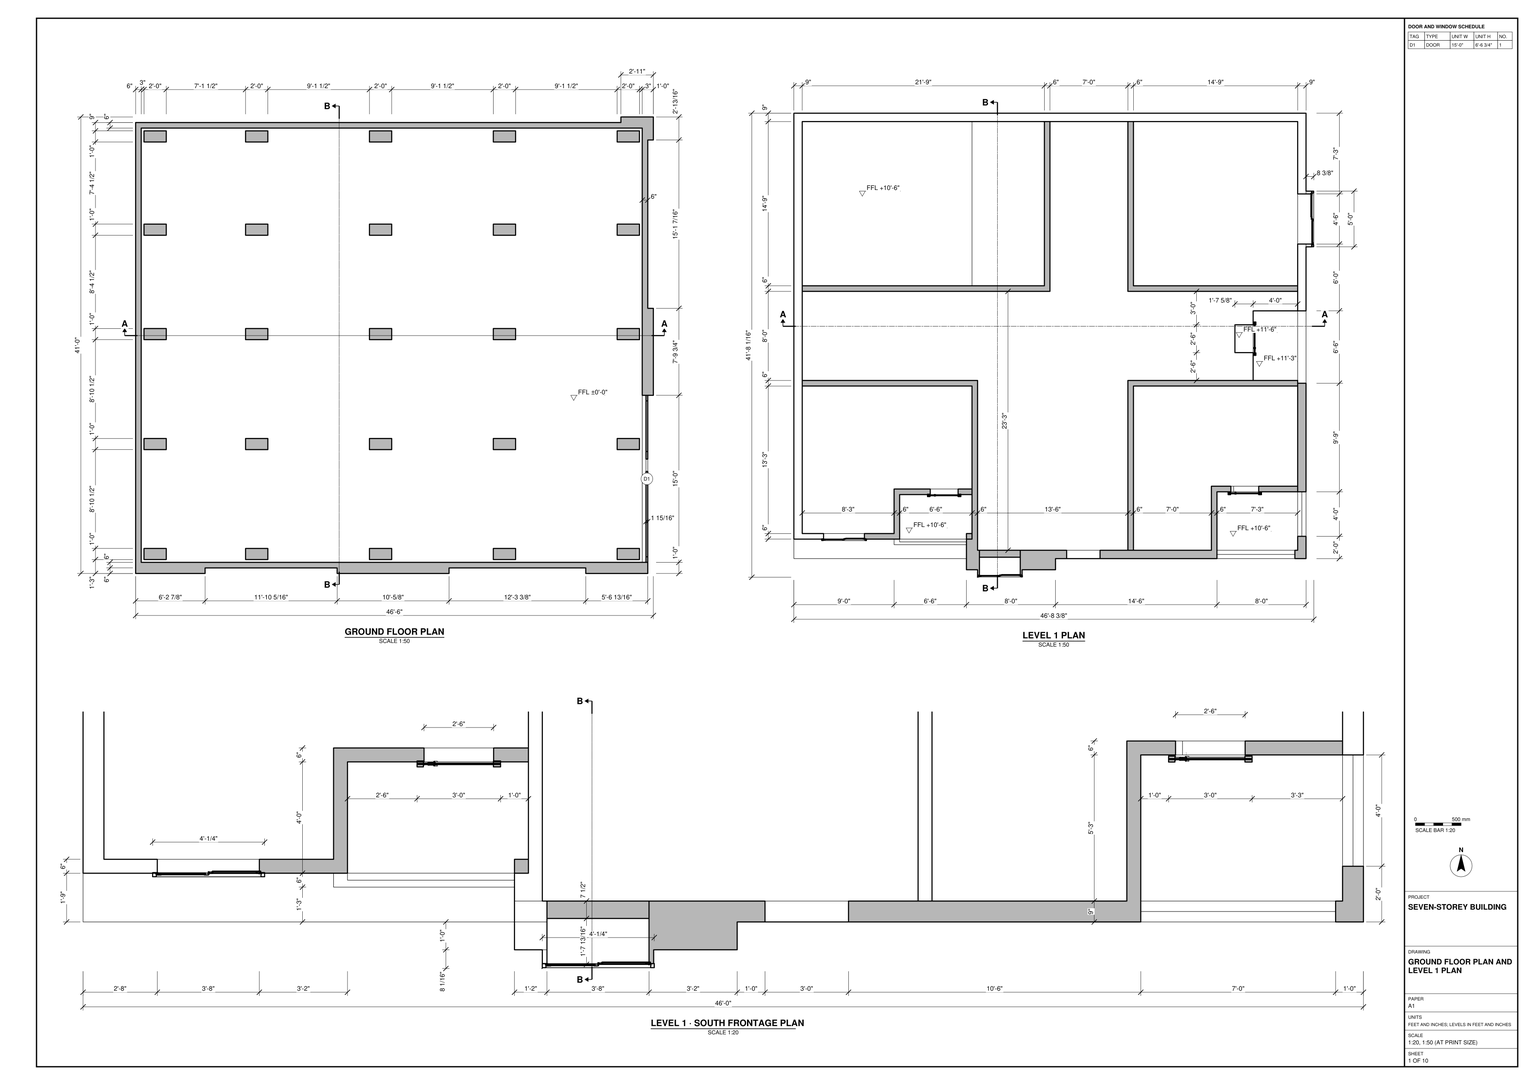
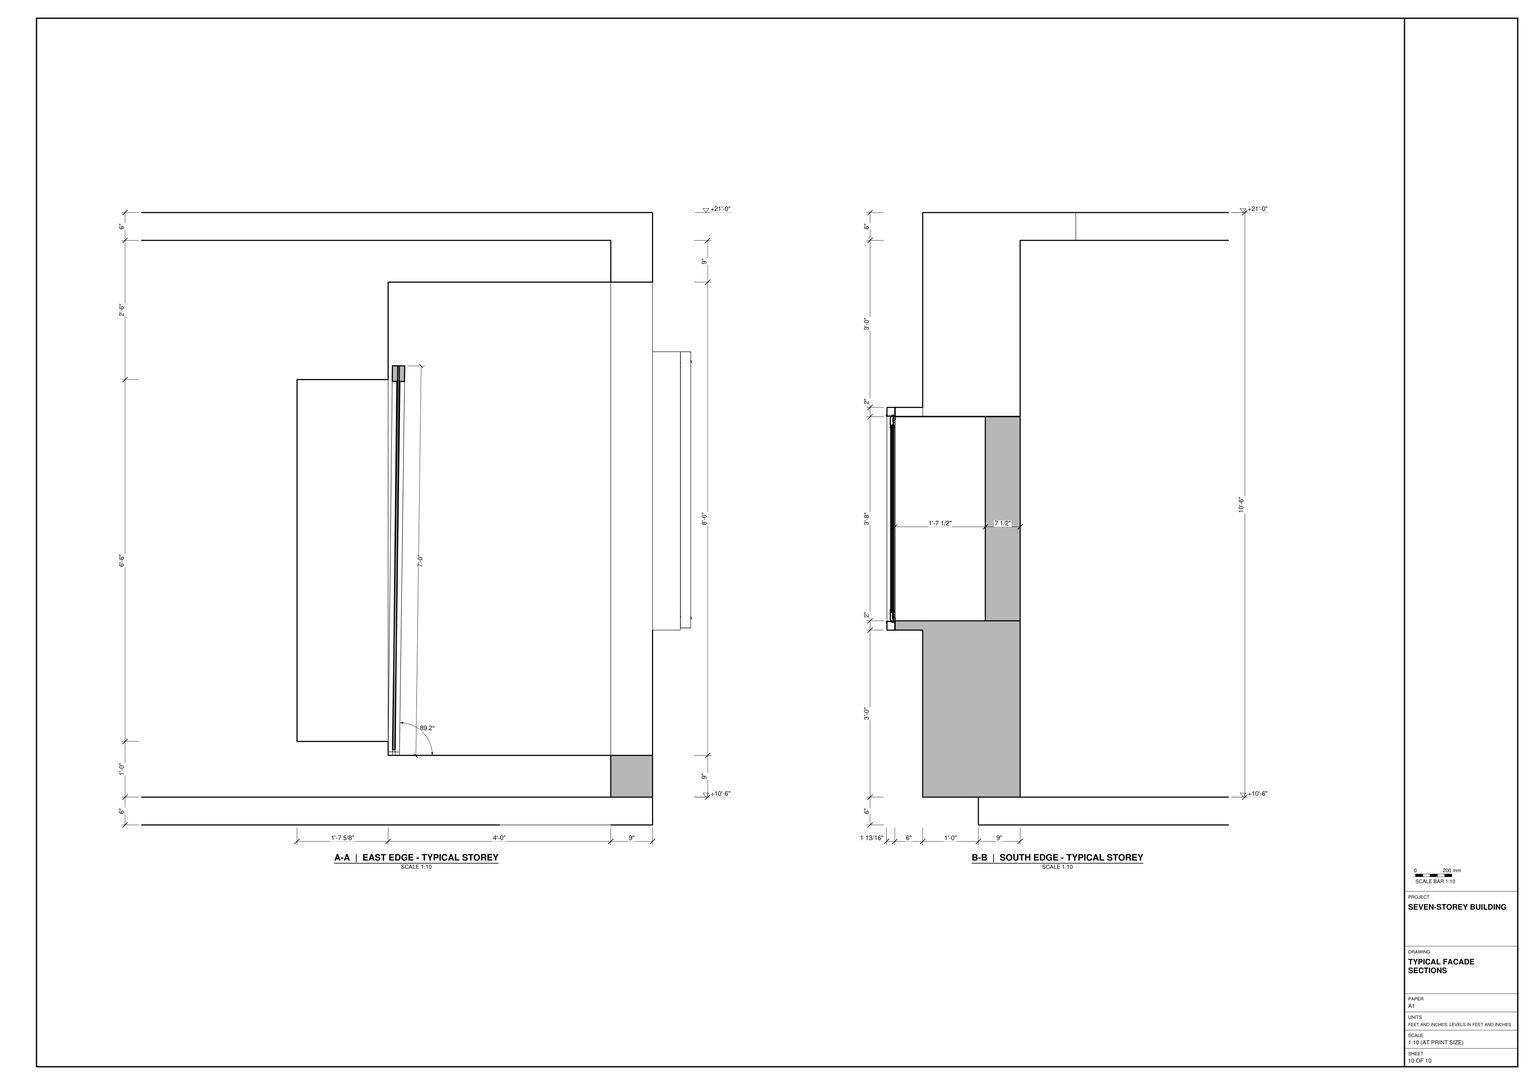
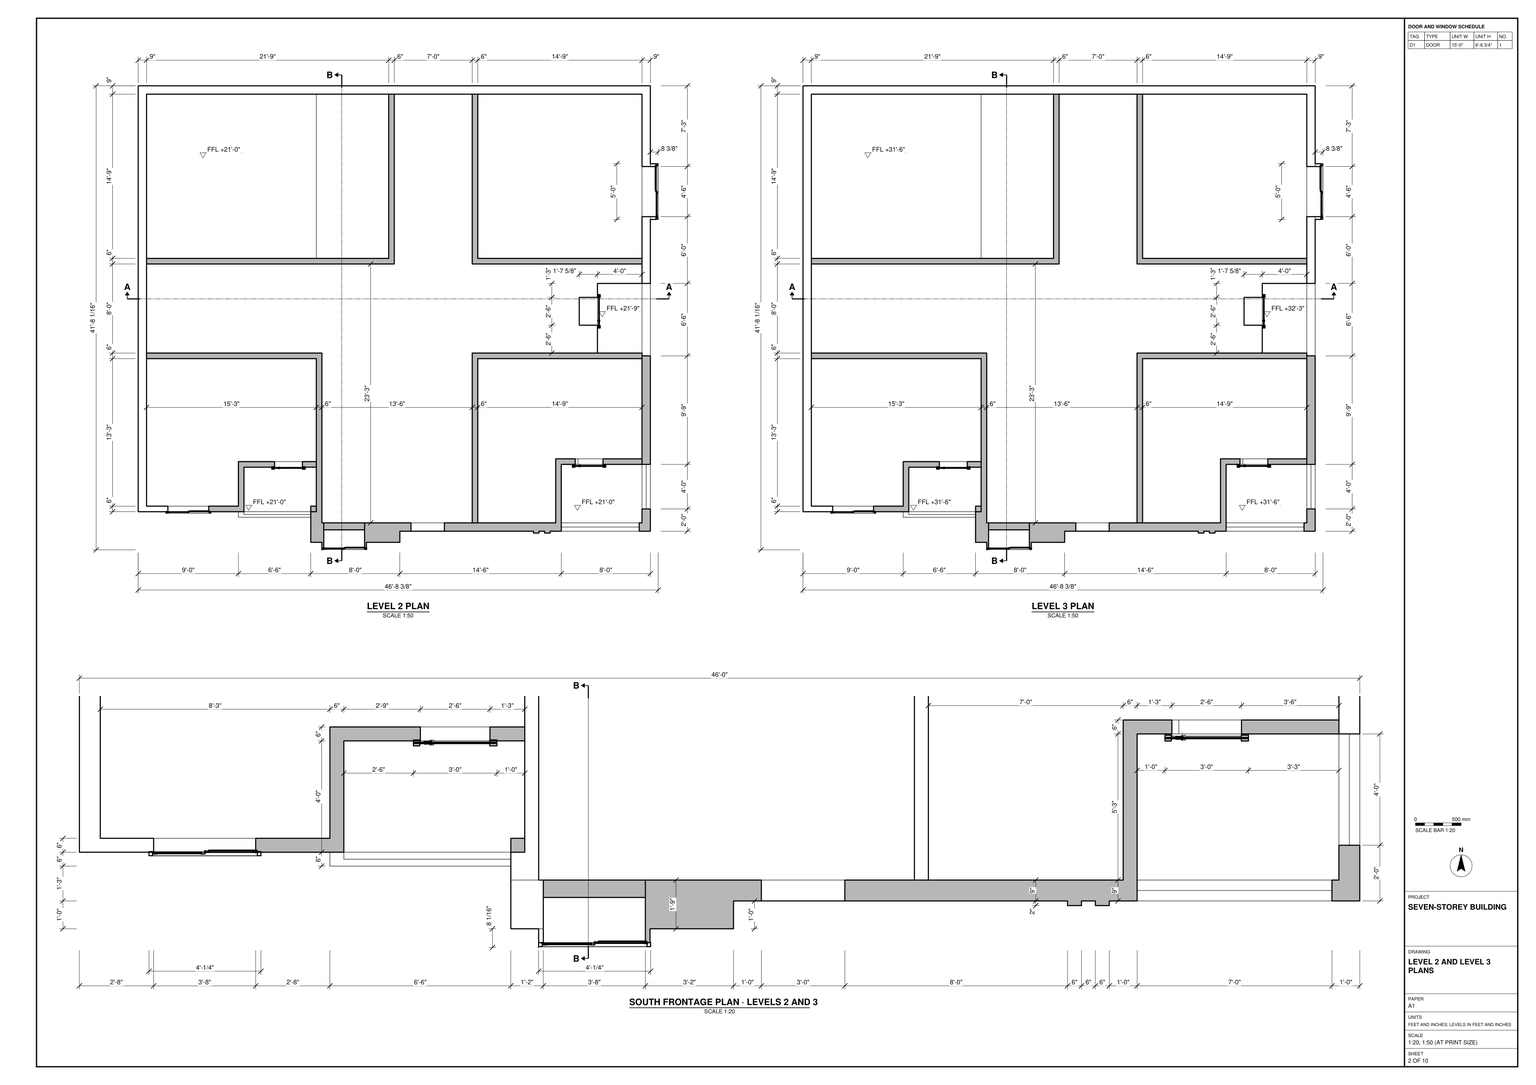
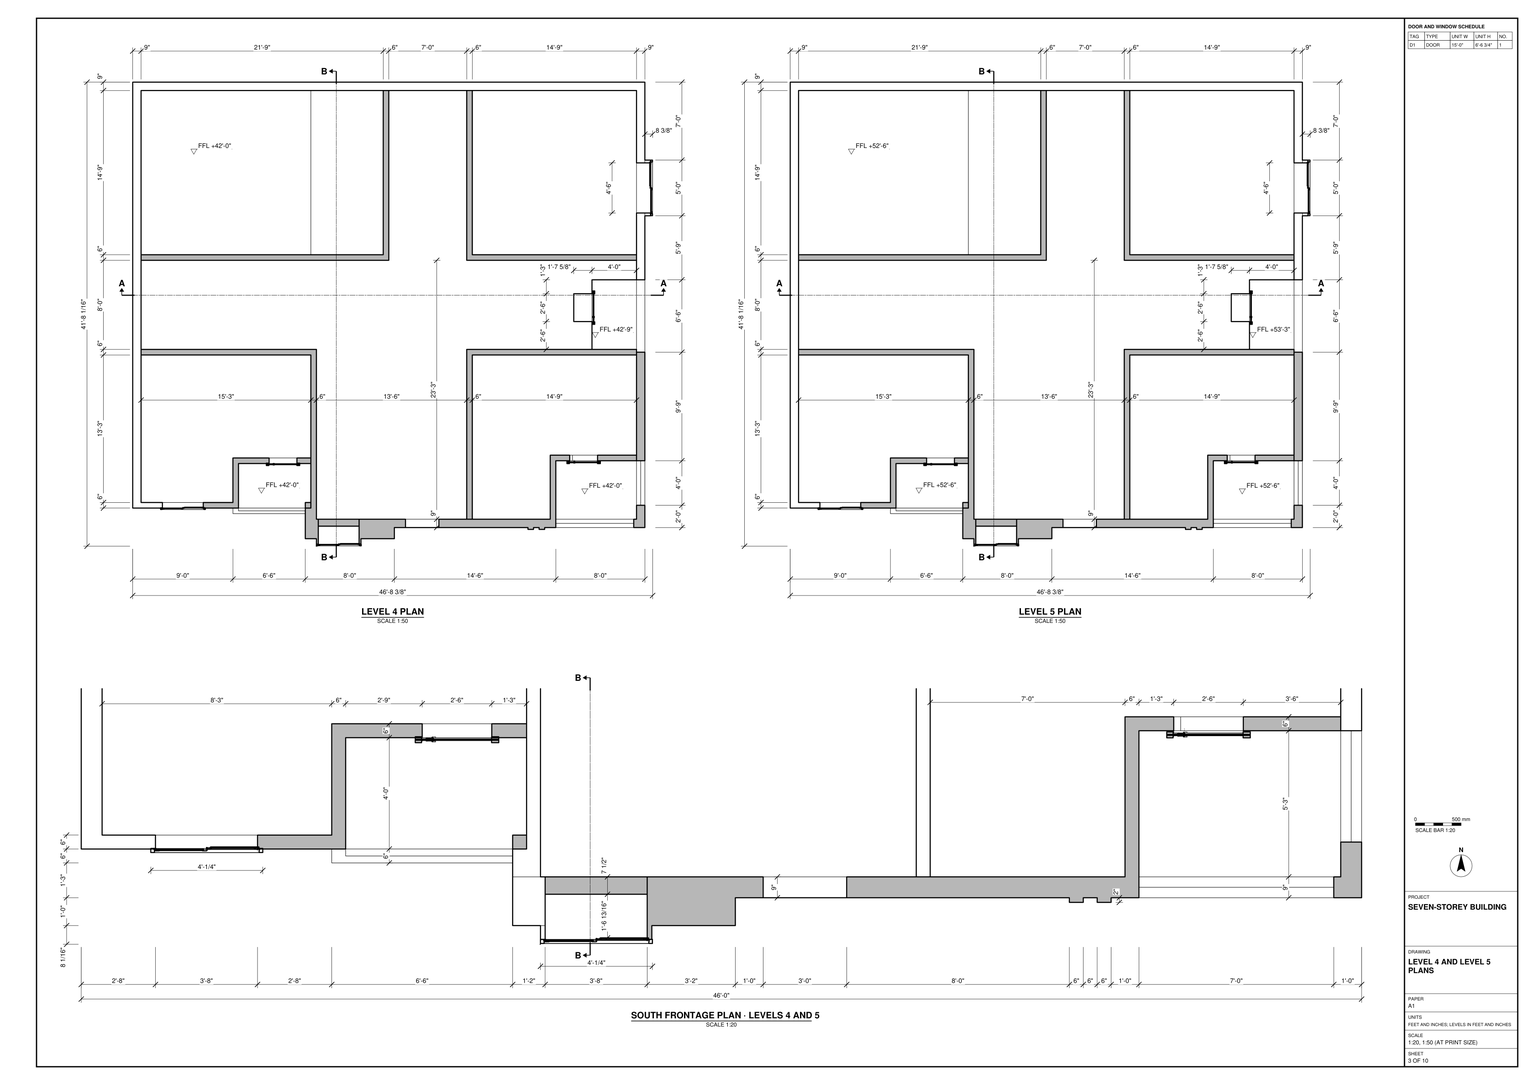
Build the seven-storey building in SketchUp from task_files/diagram_01.pdf. Work in feet and inches. The overall size, including façade projections, is 46'-8 3/8" east to west by 42'-1 13/16" north to south by 75'-0" high. Set the finished floor levels at ±0'-0", +10'-6", +21'-0", +31'-6", +42'-0", +52'-6" and +63'-0".

Start with the ground-floor perimeter, the grid of rectangular columns and the wide entrance door near the south end of the east wall. Keep the floor open between the columns. Build the upper floor slabs and walls from their respective plans, distinguishing the 9" main perimeter walls from the 6" partitions. Follow the enlarged south frontage plans for the recessed bays, wall returns and projecting window. Use the façade sections to set the openings, sills and heads in depth, not just to locate them on the wall faces. Include the changes in floor height at the east edge and finish the roof to the profile shown.

Keep walls, slabs and roof elements in separate groups or components. Keep each furniture or joinery piece shown separate and use components for repeated parts. Decor and loose items, where shown, may be any suitable library components. Save one SketchUp model as output_files/seven_storey_building_with_a_columned_ground_floor.skp.

# SketchUp Ruby script. Lengths in inches.
U = 1.inch
M = Sketchup.active_model
def pt(a) = Geom::Point3d.new(a.map { |v| v * U })
def face(e, loops, mat)
  f = e.add_face(loops[0].map { |a| pt(a) })
  loops[1..].each { |l| e.add_face(l.map { |a| pt(a) }).erase! }
  f.material = f.back_material = mat if mat
  f
end
# faces: each face lists its corners as indices into pts; further lists are holes
def faces(e, pts, list, mat = nil) = list.each { |f| face(e, (f[0].is_a?(Array) ? f : [f]).map { |l| l.map { |i| pts[i] } }, mat) }
# xy, xz, yz: faces in a plane at the given z, y or x. An outline is a flat list of corners, or four numbers for a rectangle; further outlines are holes
def ring(l) = l.size == 4 ? [[l[0], l[1]], [l[2], l[1]], [l[2], l[3]], [l[0], l[3]]] : l.each_slice(2).to_a
def flat(e, list, mat, &to3) = list.each { |f| face(e, (f[0].is_a?(Array) ? f : [f]).map { |l| ring(l).map { |u, v| to3.(u, v) } }, mat) }
def xy(e, z, list, mat = nil) = flat(e, list, mat) { |x, y| [x, y, z] }
def xz(e, y, list, mat = nil) = flat(e, list, mat) { |x, z| [x, y, z] }
def yz(e, x, list, mat = nil) = flat(e, list, mat) { |y, z| [x, y, z] }
def lines(e, pts, list) = list.each { |a, b| e.add_line(pt(pts[a]), pt(pts[b])) }
# prism: a flat outline (further loops are holes) pulled along v
def prism(e, loops, v, mat = nil)
  f = face(e, loops, mat); d = Geom::Vector3d.new(v.map { |x| x * U })
  f.pushpull(f.normal.samedirection?(d) ? d.length : -d.length)
end
def box(e, o, s, mat = nil) = prism(e, [[o, [o[0] + s[0], o[1], o[2]], [o[0] + s[0], o[1] + s[1], o[2]], [o[0], o[1] + s[1], o[2]]]], [0, 0, s[2]], mat)
def at(x, y, z, deg = 0) = Geom::Transformation.translation(pt([x, y, z])) * Geom::Transformation.rotation(ORIGIN, Z_AXIS, deg.degrees)
def axes(o, x, y, z) = Geom::Transformation.new([*x, 0, *y, 0, *z, 0, *pt(o).to_a, 1])
def part(name) = M.definitions.add(name)
# library, detail: a bought-in or finely detailed component or shape, given as its bounding box
def library(name, o, s) = part(name).tap { |d| box(d.entities, o, s) }
def detail(e, o, s) = box(e.add_group.entities, o, s)
def put(e, d, t, mat = nil) = e.add_instance(d, t).tap { |i| i.material = mat if mat }
def group(e, t, mat = nil) = e.add_group.tap { |g| g.transformation = t; g.material = mat if mat }.entities
root = M.entities
M.materials.add("Glass_Basic_01").color = [26, 26, 255]
M.materials["Glass_Basic_01"].alpha = 0.25
M.materials.add("Marble_07_1K").color = [36, 34, 36]
M.materials.add("Plaster_04_1K").color = [170, 170, 170]
M.materials.add("Plaster_04_1K1").color = [106, 98, 87]
M.materials.add("Wood_Veneer_15_1K").color = [103, 69, 45]
M.materials.add("[Color_000]").color = [255, 255, 255]
c1 = library("porta+4",[0.2,-5.42,1.33],[46.55,4.72,83.21])
c2 = library("mesh-166",[-1553.69,-2604.3125,-42.18],[1702.88,1401.6,88.28])
c3 = part("Group17")
put(c3.entities,c2,at(294.66,859.51,3.5))
c4 = part("fist floor")
p = [[270,294,120],[9,294,120],[9,471,120],[18.84,480,120],[543,471,120],[543,480,120],
  [543,9,120],[543,0,120],[543,294,120],[366,294,120],[366,471,120],[270,471,120]]
lines(c4.entities,p,[[0,1],[2,3],[4,5],[6,7],[4,8],[8,9],[10,4],[1,2],[2,11],[11,0],[9,10]])
put(c4.entities,c1,axes([467.84,73.84,-1.39],[0.77339,0,0],[0,1,0],[0,0,1.01005]))
put(c4.entities,c1,axes([493.16,218.84,7.61],[0,0.77339,0],[-1,0,0],[0,0,1.01005]))
put(c4.entities,c1,axes([143.84,71.76,-1.36],[0.77339,0,0],[0,1,0],[0,0,1.01005]))
put(c4.entities,c3,axes([65.6875,20.8,95.76],[0.02835,0,0],[0,0,0.03426],[0,-0.02835,0]))
put(c4.entities,c3,axes([413.66,-0.54,89.875],[0.01403,0,0],[0,0,0.01712],[0,-0.01389,0]))
put(c4.entities,c3,axes([558.61,380.4,110.58],[0,0.03515,0],[0,0,0.04248],[0.03515,0,0]))
put(c4.entities,c3,axes([233.68,-18.39,95.76],[0.02835,0,0],[0,0,0.03426],[0,-0.02835,0]))
put(c4.entities,c3,axes([558.54,137.6,89.8],[0,0.01398,0],[0,0,0.0169],[0.01398,0,0]))
g1 = group(c4.entities,at(0,0,0))
xy(g1,0,[[186,-12,186,9,450,9,450,78,474,78,474,72,456,72,456,0,444,0,444,-2,438,-2,438,0,432,0,432,-2,426,-2,426,0,282,0,282,-12],[456,0,456,9,543,9,543,24,552,24,552,0],[198,9,360,9,360,192,543,192,543,288,360,288,360,471,276,471,276,288,9,288,9,192,198,192],[366,9,450,9,450,78,543,78,543,186,366,186],[456,9,543,72],
  [0,21,0,480,552,480,552,24,543,24,543,471,9,471,9,27,108,27,108,75,192,75,192,69,114,69,114,21],[114,21,186,21,186,27,192,27,192,69,114,69],[186,21,192,27],[9,27,108,27,108,75,192,75,192,186,9,186],[474,72,543,78],
  [9,294,192,471],[192,294,270,471],[366,294,543,471]])
xy(g1,0.33,[[114,18,186,21]])
xy(g1,3,[[147,69,177,75],[471,72,474,78],[474,72,501,78]])
xy(g1,5.71,[[294,0,330,9]])
xy(g1,9,[[543,189,552,267],[495,192,543,267]])
xy(g1,12,[[475.36,222,495,252]])
xy(g1,24,[[456,0,540,4.5],[547.5,24,552,72]])
xy(g1,36,[[198,-18,246,-12],[456,4.5,540,9],[108,15,186,15,186,18,114,18,114,21,108,21],[543,24,547.5,72],[552,336,558,396]])
xy(g1,38,[[200,-18,244,1.5],[200,1.5,244,9],[32,21,76,27]])
xy(g1,39,[[543,339,558,393]])
xy(g1,60,[[552,120,558,144]])
xy(g1,62,[[398,0,418,9],[543,122,558,142]])
xy(g1,81,[[147,69,177,75],[471,72,501,78]])
xy(g1,82,[[200,-18,244,1.5],[398,0,418,9],[200,1.5,244,9],[32,21,76,27],[543,122,558,142]])
xy(g1,84,[[198,-18,246,-12],[552,120,558,144]])
xy(g1,90,[[475.36,222,495,252]])
xy(g1,93,[[543,339,558,393]])
xy(g1,96,[[114,21,186,27],[552,336,558,396]])
xy(g1,108,[[456,0,540,9],[543,24,552,72]])
xy(g1,111,[[543,189,552,267],[495,192,543,267]])
xy(g1,114.57,[[294,0,330,9]])
xy(g1,120,[[198,9,360,186],[360,9,366,186],[366,9,366,186,543,186,543,78,450,78,450,9],[456,9,543,72],[0,21,0,186,9,186,9,27,108,27,108,75,192,75,192,69,114,69,114,27,192,27,192,21],
  [9,27,9,186,192,186,192,75,108,75,108,27],[114,27,192,69],[474,72,543,78],[0,186,9,192],[9,186,198,192],
  [198,186,360,192],[360,186,366,192],[366,186,543,192],[0,192,9,288],[9,192,543,288],
  [0,288,9,294],[9,288,276,294],[276,288,360,294],[360,288,543,294],[0,294,9,471],
  [9,294,270,471],[270,294,276,471],[276,294,360,471],[360,294,366,471],[366,294,543,471]])
xy(g1,126,[[186,-12,282,-12,282,0,426,0,426,-2,432,-2,432,0,438,0,438,-2,444,-2,444,0,552,0,552,480,0,480,0,21,186,21]])
xz(g1,-18,[[[198,36,246,84],[200,38,244,82]]])
xz(g1,-12,[[252,0,282,126]])
xz(g1,-12,[[[186,0,252,126],[198,36,246,84]]],"Wood_Veneer_15_1K")
xz(g1,-2,[[426,0,432,126],[438,0,444,126]],"Marble_07_1K")
xz(g1,0,[[[282,0,426,126],[294,5.71,330,114.57],[396,60,420,84]],[432,0,438,126],[[444,0,552,126],[456,24,540,108]],[[396,60,420,84],[398,62,418,82]]])
xz(g1,0,[[294,5.71,330,114.57]],"Glass_Basic_01")
xz(g1,1.5,[[200,38,244,82]],"Glass_Basic_01")
xz(g1,4.5,[[456,24,540,36]],"Glass_Basic_01")
xz(g1,9,[[[198,0,360,120],[294,5.71,330,114.57],[200,38,244,82]],[360,0,366,120],[[366,0,450,120],[398,62,418,82]],[456,0,543,24],[540,24,540,108,474,108,474,120,543,120,543,24],
  [456,108,474,120]])
xz(g1,9,[[456,24,540,36],[200,38,244,82]],"Glass_Basic_01")
xz(g1,15,[[108,0.33,186,36]])
xz(g1,18,[[114,0.33,186,18],[114,18,186,36]])
xz(g1,21,[[[0,0,9,0,9,0.33,108,0.33,108,36,114,36,114,96,186,96,186,120,0,120],[30,36,78,84]],[9,0,114,0.33],[114,0,186,0.33],[186,0,192,120],[[30,36,78,84],[32,38,76,82]],
  [0,120,186,126]])
xz(g1,24,[[547.5,24,547.5,36,543,36,543,108,552,108,552,24]])
xz(g1,27,[[[9,0,108,120],[32,38,76,82]],[186,0,186,96,114,96,114,120,192,120,192,0]])
xz(g1,69,[[114,0,144,0,144,84,180,84,180,0,192,0,192,120,114,120],[[144,0,180,84],[147,3,177,81]]])
xz(g1,72,[[456,0,468,0,468,84,504,84,504,0,543,0,543,120,456,120],[[468,0,504,84],[471,3,501,81]],[547.5,24,552,24,552,108,543,108,543,36,547.5,36]])
xz(g1,75,[[[108,0,192,120],[147,3,177,81]]])
xz(g1,78,[[450,0,450,120,543,120,543,0,480,0,480,3,501,3,501,81,471,81,471,3,474,3,474,0],[474,0,480,3]])
xz(g1,120,[[552,60,558,84]])
xz(g1,122,[[543,62,558,82]])
xz(g1,142,[[543,62,558,82]])
xz(g1,144,[[552,60,558,84]])
xz(g1,186,[[9,0,192,120],[366,0,543,120]])
xz(g1,189,[[543,9,552,111]])
xz(g1,192,[[9,0,198,120],[360,0,366,120],[366,0,366,120,543,120,543,111,495,111,495,9,543,9,543,0],[495,9,543,111]])
xz(g1,222,[[475.36,12,495,90]])
xz(g1,252,[[475.36,12,495,90]])
xz(g1,267,[[495,9,543,111],[543,9,552,111]])
xz(g1,288,[[9,0,276,120],[360,0,543,120]])
xz(g1,294,[[9,0,191.78,120],[191.78,0,192,120],[192,0,270,120],[366,0,543,120]])
xz(g1,336,[[552,36,558,96]])
xz(g1,339,[[543,39,558,93]])
xz(g1,393,[[543,39,558,93]])
xz(g1,396,[[552,36,558,96]])
xz(g1,471,[[9,0,270,120],[270,0,276,120],[276,0,360,120],[360,0,366,120],[366,0,543,120]])
xz(g1,480,[[0,0,552,126]])
yz(g1,0,[[21,0,480,120],[21,120,480,126]])
yz(g1,9,[[27,0,186,120],[186,0,192,120],[192,0,288,120],[288,0,294,120],[294,0,471,120]])
yz(g1,32,[[21,38,27,82]])
yz(g1,76,[[21,38,27,82]])
yz(g1,108,[[27,0,75,96],[15,0.33,21,36],[27,96,75,120]])
yz(g1,114,[[21,0,69,0,69,120,27,120,27,96,21,96],[18,0.33,21,18],[18,18,21,36]])
yz(g1,147,[[69,3,75,81]])
yz(g1,177,[[69,3,75,81]])
yz(g1,186,[[21,0,27,18],[15,0.33,18,36],[18,0.33,21,18],[18,18,21,36],[21,18,27,96]])
yz(g1,186,[[-12,0,-12,126,21,126,21,36,15,36,15,0.33,9,0.33,9,0]],"Wood_Veneer_15_1K")
yz(g1,192,[[21,0,27,120],[27,0,69,120],[69,0,75,120],[75,0,186,120]])
yz(g1,198,[[9,0,192,120],[-18,36,-12,84]])
yz(g1,200,[[-18,38,1.5,82],[1.5,38,9,82]])
yz(g1,244,[[-18,38,1.5,82],[1.5,38,9,82]])
yz(g1,246,[[-18,36,-12,84]])
yz(g1,270,[[294,0,471,120]])
yz(g1,276,[[288,0,471,120]])
yz(g1,282,[[-12,0,0,126]])
yz(g1,294,[[0,5.71,9,114.57]])
yz(g1,330,[[0,5.71,9,114.57]])
yz(g1,360,[[9,0,192,120],[288,0,471,120]])
yz(g1,366,[[9,0,186,120],[294,0,471,120]])
yz(g1,398,[[0,62,9,82]])
yz(g1,418,[[0,62,9,82]])
yz(g1,426,[[-2,0,0,126]],"Marble_07_1K")
yz(g1,432,[[-2,0,0,126]],"Marble_07_1K")
yz(g1,438,[[-2,0,0,126]],"Marble_07_1K")
yz(g1,444,[[-2,0,0,126]],"Marble_07_1K")
yz(g1,450,[[9,0,78,108],[9,108,78,120]])
yz(g1,456,[[9,0,72,0,72,120,9,120,9,108,0,108,0,24,4.5,24,4.5,36,9,36]])
yz(g1,471,[[72,3,78,81]])
yz(g1,475.36,[[222,12,252,90]])
yz(g1,495,[[192,9,219,9,219,93,255,93,255,9,267,9,267,111,192,111],[[219,9,255,93],[222,12,252,90]]])
yz(g1,501,[[72,3,78,81]])
yz(g1,540,[[0,24,0,108,9,108,9,36,4.5,36,4.5,24]])
yz(g1,543,[[9,0,9,120,72,120,72,108,24,108,24,0],[24,0,72,24],[72,0,78,120],[[78,0,186,120],[122,62,142,82]],[186,0,186,120,192,120,192,111,189,111,189,9,192,9,192,0],
  [192,0,192,9,267,9,267,111,192,111,192,120,288,120,288,0],[288,0,294,120],[[294,0,471,120],[339,39,393,93]],[189,9,192,111]])
yz(g1,543,[[24,24,72,36]],"Glass_Basic_01")
yz(g1,547.5,[[24,24,72,36]],"Glass_Basic_01")
yz(g1,552,[[[0,0,180,120],[24,24,72,108],[120,60,144,84]],[[180,0,276,120],[189,9,267,111]],[0,120,480,126]])
yz(g1,552,[[189,9,267,36]],"Glass_Basic_01")
yz(g1,552,[[276,0,480,12],[276,12,480,24],[276,24,480,36],[276,36,336,48],[396,36,480,48],
  [276,48,336,60],[396,48,480,60],[276,60,336,72],[396,60,480,72],[276,72,336,84],
  [396,72,480,84],[276,84,336,96],[396,84,480,96],[276,96,480,108],[276,108,480,120]],"Wood_Veneer_15_1K")
yz(g1,558,[[[336,36,396,96],[339,39,393,93]],[[120,60,144,84],[122,62,142,82]]])
p = [[186,9,120],[198,9,120]]
lines(g1,p,[[0,1]])
c5 = library("Modern+Gate+1",[0,0,0],[118.11,1.97,78.74])
box(root,[192,12,756],[54,66,102])
xy(root,-6,[[0,12,0,498,523.03,498,523.03,504,558,504,558,479.1875,552,479.1875,552,297.76,558,297.76,558,204,552,204,552,27,543,27,543,12,485.17,12,485.17,18,337.78,18,337.78,12,217.17,12,217.17,18,74.85,18,74.85,12],[543,12,552,27]])
xy(root,0,[[[6,24,546,492],[9,264,33,276],[9,376.5,33,388.5],[118.5,376.5,142.5,388.5],[9,477,33,489],[118.5,477,142.5,489],[252,477,276,489],[252,376.5,276,388.5],[385.5,477,409.5,489],[385.5,376.5,409.5,388.5],[519,477,543,489],[519,376.5,543,388.5],[519,264,543,276],[385.5,264,409.5,276],[252,264,276,276],[118.5,264,142.5,276],[252,145.5,276,157.5],[385.5,145.5,409.5,157.5],[519,145.5,543,157.5],[118.5,145.5,142.5,157.5],[9,145.5,33,157.5],[385.5,27,409.5,39],[252,27,276,39],[118.5,27,142.5,39],[9,27,33,39],[519,27,543,39]],[546,24,552,204],[9,27,33,39],[519,27,543,39]])
xy(root,72,[[0,12,74.85,12,74.85,18,217.17,18,217.17,12,337.78,12,337.78,18,485.17,18,485.17,12,552,12,552,24,0,24],[0,24,6,24,6,492,546,492,546,204,558,204,558,297.76,552,297.76,552,479.1875,558,479.1875,558,504,523.03,504,523.03,498,0,498]])
xy(root,120,[[[0,18,552,498],[9,27,543,489]],[33,27,33,39,9,39,9,145.5,142.5,145.5,142.5,39,118.5,39,118.5,27],[142.5,27,142.5,145.5,276,145.5,276,39,252,39,252,27],[276,27,276,145.5,409.5,145.5,409.5,39,385.5,39,385.5,27],[409.5,27,409.5,145.5,543,145.5,543,39,519,39,519,27],
  [33,145.5,33,157.5,9,157.5,9,264,142.5,264,142.5,157.5,118.5,157.5,118.5,145.5],[142.5,145.5,142.5,264,276,264,276,157.5,252,157.5,252,145.5],[276,145.5,276,264,409.5,264,409.5,157.5,385.5,157.5,385.5,145.5],[409.5,145.5,409.5,264,543,264,543,157.5,519,157.5,519,145.5],[33,264,33,276,9,276,9,376.5,142.5,376.5,142.5,276,118.5,276,118.5,264],
  [142.5,264,142.5,376.5,276,376.5,276,276,252,276,252,264],[276,264,276,376.5,409.5,376.5,409.5,276,385.5,276,385.5,264],[409.5,264,409.5,376.5,543,376.5,543,276,519,276,519,264],[33,376.5,33,388.5,9,388.5,9,477,33,477,33,489,118.5,489,118.5,477,142.5,477,142.5,388.5,118.5,388.5,118.5,376.5],[142.5,376.5,142.5,489,252,489,252,477,276,477,276,388.5,252,388.5,252,376.5],
  [276,376.5,276,489,385.5,489,385.5,477,409.5,477,409.5,388.5,385.5,388.5,385.5,376.5],[409.5,376.5,409.5,489,519,489,519,477,543,477,543,388.5,519,388.5,519,376.5]])
xy(root,126,[[0,18,543,18,543,27,552,27,552,498,0,498],[543,18,552,27]])
xy(root,630,[[186,6,186,27,450,27,450,96,474,96,474,90,456,90,456,18,444,18,444,16,438,16,438,18,432,18,432,16,426,16,426,18,282,18,282,6],[456,18,456,27,543,27,543,42,552,42,552,18],[198,27,360,27,360,210,543,210,543,306,360,306,360,489,276,489,276,306,9,306,9,210,198,210],[366,27,450,27,450,96,543,96,543,204,366,204],[456,27,543,90],
  [0,39,0,498,552,498,552,42,543,42,543,489,9,489,9,45,108,45,108,93,192,93,192,87,114,87,114,39],[114,39,186,39,186,45,192,45,192,87,114,87],[186,39,192,45],[9,45,108,45,108,93,192,93,192,204,9,204],[474,90,543,96],
  [9,312,192,489],[192,312,270,489],[366,312,543,489]])
xy(root,630.33,[[114,36,186,39]])
xy(root,633,[[147,87,177,93],[471,90,474,96],[474,90,501,96]])
xy(root,635.71,[[294,18,330,27]])
xy(root,639,[[543,207,552,285],[495,210,543,285]])
xy(root,642,[[475.36,240,495,270]])
xy(root,654,[[456,18,540,22.5],[547.5,42,552,90]])
xy(root,666,[[198,0,246,6],[456,22.5,540,27],[108,33,186,33,186,36,114,36,114,39,108,39],[543,42,547.5,90],[552,354,558,414]])
xy(root,668,[[200,0,244,19.5],[200,19.5,244,27],[32,39,76,45]])
xy(root,669,[[543,357,558,411]])
xy(root,690,[[552,138,558,162]])
xy(root,692,[[398,18,418,27],[543,140,558,160]])
xy(root,711,[[147,87,177,93],[471,90,501,96]])
xy(root,712,[[200,0,244,19.5],[398,18,418,27],[200,19.5,244,27],[32,39,76,45],[543,140,558,160]])
xy(root,714,[[198,0,246,6],[552,138,558,162]])
xy(root,720,[[475.36,240,495,270]])
xy(root,723,[[543,357,558,411]])
xy(root,726,[[114,39,186,45],[552,354,558,414]])
xy(root,738,[[456,18,540,27],[543,42,552,90]])
xy(root,741,[[543,207,552,285],[495,210,543,285]])
xy(root,744.57,[[294,18,330,27]])
xy(root,750,[[426,16,432,18],[438,16,444,18],[543,18,552,498],[198,27,360,204],[360,27,366,204],
  [366,27,366,204,543,204,543,96,450,96,450,27],[456,27,474,90],[474,27,543,90],[0,39,0,204,9,204,9,45,108,45,108,93,192,93,192,87,114,87,114,45,192,45,192,39],[9,45,9,204,192,204,192,93,108,93,108,45],
  [114,45,192,87],[474,90,543,96],[0,204,9,210],[9,204,198,210],[198,204,360,210],
  [360,204,366,210],[366,204,543,210],[0,210,9,306],[9,210,543,306],[0,306,9,312],
  [9,306,276,312],[276,306,360,312],[360,306,543,312],[0,312,9,489],[9,312,270,489],
  [270,312,276,489],[276,312,360,489],[360,312,366,489],[366,312,543,489],[0,489,0,498,18.84,498,9,489],
  [9,489,18.84,498,543,498,543,489]])
xy(root,756,[[252,12,276,12,276,30,378,30,378,24,546,24,546,492,6,492,6,45,186,45,186,84,252,84]])
xy(root,792,[[252,6,282,6,282,30,276,30,276,12,252,12],[378,18,546,24],[0,39,186,39,186,45,6,45,6,492,492,492,492,498,0,498],[546,42,552,492],[492,492,552,498]])
xy(root,858,[[182,2,256,6],[182,6,186,39],[252,6,256,88],[182,39,186,45],[182,45,186,88],
  [186,84,192,88],[192,84,252,88]])
xy(root,864,[[182,2,256,88]])
xy(root,888,[[282,18,378,30],[[378,18,378,30,282,30,282,42,492,42,492,492,552,492,552,42,546,42,546,18],[504,474.6,540,486],[504,87,540,98.4],[504,109.8,540,121.2],[504,132.6,540,144],[504,178.2,540,189.6],[504,201,540,212.4],[504,269.4,540,280.8],[504,292.2,540,303.6],[504,315,540,326.4],[504,337.8,540,349.2],[504,360.6,540,372],[504,383.4,540,394.8],[504,406.2,540,417.6],[504,429,540,440.4],[504,451.8,540,463.2],[504,41.4,540,52.8],[504,64.2,540,75.6],[504,155.4,540,166.8],[504,223.8,540,235.2],[504,246.6,540,258]],[546,18,552,24],[546,24,552,42]])
xy(root,894,[[282,18,492,42],[[492,18,552,498],[504,41.4,540,486]],[504,52.8,540,64.2],[504,75.6,540,87],[504,98.4,540,109.8],
  [504,121.2,540,132.6],[504,144,540,155.4],[504,166.8,540,178.2],[504,189.6,540,201],[504,212.4,540,223.8],
  [504,235.2,540,246.6],[504,258,540,269.4],[504,280.8,540,292.2],[504,303.6,540,315],[504,326.4,540,337.8],
  [504,349.2,540,360.6],[504,372,540,383.4],[504,394.8,540,406.2],[504,417.6,540,429],[504,440.4,540,451.8],
  [504,463.2,540,474.6]])
xz(root,0,[[[198,666,246,714],[200,668,244,712]]])
xz(root,2,[[182,858,256,864]])
xz(root,6,[[252,630,282,792]])
xz(root,6,[[[186,630,252,858],[198,666,246,714]]],"Wood_Veneer_15_1K")
xz(root,12,[[0,-6,74.85,72],[217.17,-6,337.78,72],[485.17,-6,552,72],[252,756,276,792]])
xz(root,16,[[426,630,432,750],[438,630,444,750]],"Marble_07_1K")
xz(root,18,[[0,120,552,126],[[282,630,426,750],[294,635.71,330,744.57],[396,690,420,714]],[432,630,438,750],[[444,630,552,750],[456,654,540,738]],[[396,690,420,714],[398,692,418,712]],
  [282,750,378,888],[546,792,552,888],[282,888,552,894]])
xz(root,18,[[294,635.71,330,744.57]],"Glass_Basic_01")
xz(root,18,[[102.66,-6,217.17,30.46],[337.78,-6,451.57,33.19]],"Plaster_04_1K1")
xz(root,18,[[74.85,-6,102.66,-6,102.66,30.46,217.17,30.46,217.17,72,74.85,72],[451.57,-6,485.17,-6,485.17,72,337.78,72,337.78,33.19,451.57,33.19],[378,750,552,790]],"Wood_Veneer_15_1K")
xz(root,18,[[378,790,552,792]],"[Color_000]")
xz(root,19.5,[[200,668,244,712]],"Glass_Basic_01")
xz(root,22.5,[[456,654,540,666]],"Glass_Basic_01")
xz(root,24,[[6,0,546,72],[546,0,552,72],[378,756,426,792],[426,756,432,792],[432,756,438,792],
  [438,756,444,792],[444,756,546,792]])
xz(root,27,[[9,0,33,120],[118.5,0,142.5,120],[252,0,276,120],[385.5,0,409.5,120],[519,0,543,120],
  [[198,630,360,750],[294,635.71,330,744.57],[200,668,244,712]],[360,630,366,750],[[366,630,450,750],[398,692,418,712]],[456,630,543,654],[540,654,540,738,474,738,474,750,543,750,543,654],
  [456,738,474,750]])
xz(root,27,[[456,654,540,666],[200,668,244,712]],"Glass_Basic_01")
xz(root,30,[[276,756,276,792,282,792,282,888,378,888,378,756]])
xz(root,33,[[108,630.33,186,666]])
xz(root,36,[[114,630.33,186,648],[114,648,186,666]])
xz(root,39,[[9,0,33,120],[118.5,0,142.5,120],[252,0,276,120],[385.5,0,409.5,120],[519,0,543,120],
  [[0,630,9,630,9,630.33,108,630.33,108,666,114,666,114,726,186,726,186,750,0,750],[30,666,78,714]],[9,630,114,630.33],[114,630,186,630.33],[186,630,192,750],[[30,666,78,714],[32,668,76,712]]])
xz(root,39,[[0,750,186,792]],"Wood_Veneer_15_1K")
xz(root,41.4,[[504,888,540,894]])
xz(root,42,[[547.5,654,547.5,666,543,666,543,738,552,738,552,654],[546,792,552,888],[282,888,492,894]])
xz(root,45,[[[9,630,108,750],[32,668,76,712]],[186,630,186,726,114,726,114,750,192,750,192,630],[6,756,186,792]])
xz(root,52.8,[[504,888,540,894]])
xz(root,64.2,[[504,888,540,894]])
xz(root,75.6,[[504,888,540,894]])
xz(root,84,[[186,756,252,858]],"Wood_Veneer_15_1K")
xz(root,87,[[114,630,144,630,144,714,180,714,180,630,192,630,192,750,114,750],[[144,630,180,714],[147,633,177,711]],[504,888,540,894]])
xz(root,88,[[182,858,256,864]])
xz(root,90,[[456,630,468,630,468,714,504,714,504,630,543,630,543,750,456,750],[[468,630,504,714],[471,633,501,711]],[547.5,654,552,654,552,738,543,738,543,666,547.5,666]])
xz(root,93,[[[108,630,192,750],[147,633,177,711]]])
xz(root,96,[[450,630,450,750,543,750,543,630,480,630,480,633,501,633,501,711,471,711,471,633,474,633,474,630],[474,630,480,633]])
xz(root,98.4,[[504,888,540,894]])
xz(root,109.8,[[504,888,540,894]])
xz(root,121.2,[[504,888,540,894]])
xz(root,132.6,[[504,888,540,894]])
xz(root,138,[[552,690,558,714]])
xz(root,140,[[543,692,558,712]])
xz(root,144,[[504,888,540,894]])
xz(root,145.5,[[9,0,33,120],[118.5,0,142.5,120],[252,0,276,120],[385.5,0,409.5,120],[519,0,543,120]])
xz(root,155.4,[[504,888,540,894]])
xz(root,157.5,[[9,0,33,120],[118.5,0,142.5,120],[252,0,276,120],[385.5,0,409.5,120],[519,0,543,120]])
xz(root,160,[[543,692,558,712]])
xz(root,162,[[552,690,558,714]])
xz(root,166.8,[[504,888,540,894]])
xz(root,178.2,[[504,888,540,894]])
xz(root,189.6,[[504,888,540,894]])
xz(root,201,[[504,888,540,894]])
xz(root,204,[[552,-6,558,0],[546,0,558,72],[9,630,192,750],[366,630,543,750]])
xz(root,207,[[543,639,552,741]])
xz(root,210,[[9,630,198,750],[360,630,366,750],[366,630,366,750,543,750,543,741,495,741,495,639,543,639,543,630],[495,639,543,741]])
xz(root,212.4,[[504,888,540,894]])
xz(root,223.8,[[504,888,540,894]])
xz(root,235.2,[[504,888,540,894]])
xz(root,240,[[475.36,642,495,720]])
xz(root,246.6,[[504,888,540,894]])
xz(root,258,[[504,888,540,894]])
xz(root,264,[[9,0,33,120],[118.5,0,142.5,120],[252,0,276,120],[385.5,0,409.5,120],[519,0,543,120]])
xz(root,269.4,[[504,888,540,894]])
xz(root,270,[[475.36,642,495,720]])
xz(root,276,[[9,0,33,120],[118.5,0,142.5,120],[252,0,276,120],[385.5,0,409.5,120],[519,0,543,120]])
xz(root,280.8,[[504,888,540,894]])
xz(root,285,[[495,639,543,741],[543,639,552,741]])
xz(root,292.2,[[504,888,540,894]])
xz(root,297.76,[[552,-6,558,72]])
xz(root,303.6,[[504,888,540,894]])
xz(root,306,[[9,630,276,750],[360,630,543,750]])
xz(root,312,[[9,630,191.78,750],[191.78,630,192,750],[192,630,270,750],[366,630,543,750]])
xz(root,315,[[504,888,540,894]])
xz(root,326.4,[[504,888,540,894]])
xz(root,337.8,[[504,888,540,894]])
xz(root,349.2,[[504,888,540,894]])
xz(root,354,[[552,666,558,726]])
xz(root,357,[[543,669,558,723]])
xz(root,360.6,[[504,888,540,894]])
xz(root,372,[[504,888,540,894]])
xz(root,376.5,[[9,0,33,120],[118.5,0,142.5,120],[252,0,276,120],[385.5,0,409.5,120],[519,0,543,120]])
xz(root,383.4,[[504,888,540,894]])
xz(root,388.5,[[9,0,33,120],[118.5,0,142.5,120],[252,0,276,120],[385.5,0,409.5,120],[519,0,543,120]])
xz(root,394.8,[[504,888,540,894]])
xz(root,406.2,[[504,888,540,894]])
xz(root,411,[[543,669,558,723]])
xz(root,414,[[552,666,558,726]])
xz(root,417.6,[[504,888,540,894]])
xz(root,429,[[504,888,540,894]])
xz(root,440.4,[[504,888,540,894]])
xz(root,451.8,[[504,888,540,894]])
xz(root,463.2,[[504,888,540,894]])
xz(root,474.6,[[504,888,540,894]])
xz(root,477,[[9,0,33,120],[118.5,0,142.5,120],[252,0,276,120],[385.5,0,409.5,120],[519,0,543,120]])
xz(root,479.1875,[[552,-6,558,72]])
xz(root,486,[[504,888,540,894]])
xz(root,489,[[9,0,33,120],[118.5,0,142.5,120],[252,0,276,120],[385.5,0,409.5,120],[519,0,543,120],
  [9,630,270,750],[270,630,276,750],[276,630,360,750],[360,630,366,750],[366,630,543,750]])
xz(root,492,[[6,0,546,72],[6,756,546,792],[492,792,552,888]])
xz(root,498,[[0,-6,523.03,72],[0,120,552,126],[0,630,552,750],[492,792,552,894]])
xz(root,498,[[0,750,552,792]],"Wood_Veneer_15_1K")
xz(root,504,[[523.03,-6,558,72]])
yz(root,0,[[12,-6,498,72],[18,120,498,126],[39,630,498,750]])
yz(root,0,[[39,750,498,792]],"Wood_Veneer_15_1K")
yz(root,6,[[24,0,492,72],[45,756,492,792]])
yz(root,9,[[27,0,39,120],[145.5,0,157.5,120],[264,0,276,120],[376.5,0,388.5,120],[477,0,489,120],
  [45,630,204,750],[204,630,210,750],[210,630,306,750],[306,630,312,750],[312,630,489,750]])
yz(root,32,[[39,668,45,712]])
yz(root,33,[[27,0,39,120],[145.5,0,157.5,120],[264,0,276,120],[376.5,0,388.5,120],[477,0,489,120]])
yz(root,74.85,[[12,-6,18,72]])
yz(root,76,[[39,668,45,712]])
yz(root,108,[[45,630,93,726],[33,630.33,39,666],[45,726,93,750]])
yz(root,114,[[39,630,87,630,87,750,45,750,45,726,39,726],[36,630.33,39,648],[36,648,39,666]])
yz(root,118.5,[[27,0,39,120],[145.5,0,157.5,120],[264,0,276,120],[376.5,0,388.5,120],[477,0,489,120]])
yz(root,142.5,[[27,0,39,120],[145.5,0,157.5,120],[264,0,276,120],[376.5,0,388.5,120],[477,0,489,120]])
yz(root,147,[[87,633,93,711]])
yz(root,177,[[87,633,93,711]])
yz(root,182,[[2,858,88,864]])
yz(root,186,[[39,630,45,648],[33,630.33,36,666],[36,630.33,39,648],[36,648,39,666],[39,648,45,726]])
yz(root,186,[[6,630,6,858,84,858,84,756,45,756,45,792,39,792,39,666,33,666,33,630.33,27,630.33,27,630]],"Wood_Veneer_15_1K")
yz(root,192,[[39,630,45,750],[45,630,87,750],[87,630,93,750],[93,630,204,750]])
yz(root,198,[[27,630,210,750],[0,666,6,714]])
yz(root,200,[[0,668,19.5,712],[19.5,668,27,712]])
yz(root,217.17,[[12,-6,18,72]])
yz(root,244,[[0,668,19.5,712],[19.5,668,27,712]])
yz(root,246,[[0,666,6,714]])
yz(root,252,[[27,0,39,120],[145.5,0,157.5,120],[264,0,276,120],[376.5,0,388.5,120],[477,0,489,120]])
yz(root,252,[[12,756,84,756,84,858,6,858,6,792,12,792]],"Wood_Veneer_15_1K")
yz(root,256,[[2,858,88,864]])
yz(root,270,[[312,630,489,750]])
yz(root,276,[[27,0,39,120],[145.5,0,157.5,120],[264,0,276,120],[376.5,0,388.5,120],[477,0,489,120],
  [306,630,489,750],[12,756,30,792]])
yz(root,282,[[6,630,18,792],[18,792,30,888],[18,888,42,894]])
yz(root,294,[[18,635.71,27,744.57]])
yz(root,330,[[18,635.71,27,744.57]])
yz(root,337.78,[[12,-6,18,72]])
yz(root,360,[[27,630,210,750],[306,630,489,750]])
yz(root,366,[[27,630,204,750],[312,630,489,750]])
yz(root,378,[[24,756,30,792],[18,792,30,888]])
yz(root,385.5,[[27,0,39,120],[145.5,0,157.5,120],[264,0,276,120],[376.5,0,388.5,120],[477,0,489,120]])
yz(root,398,[[18,692,27,712]])
yz(root,409.5,[[27,0,39,120],[145.5,0,157.5,120],[264,0,276,120],[376.5,0,388.5,120],[477,0,489,120]])
yz(root,418,[[18,692,27,712]])
yz(root,426,[[16,630,18,750]],"Marble_07_1K")
yz(root,432,[[16,630,18,750]],"Marble_07_1K")
yz(root,438,[[16,630,18,750]],"Marble_07_1K")
yz(root,444,[[16,630,18,750]],"Marble_07_1K")
yz(root,450,[[27,630,96,738],[27,738,96,750]])
yz(root,456,[[27,630,90,630,90,738,18,738,18,654,22.5,654,22.5,666,27,666],[27,738,90,750]])
yz(root,471,[[90,633,96,711]])
yz(root,475.36,[[240,642,270,720]])
yz(root,485.17,[[12,-6,18,72]])
yz(root,492,[[492,792,492,888,42,888,42,894,498,894,498,792]])
yz(root,495,[[210,639,237,639,237,723,273,723,273,639,285,639,285,741,210,741],[[237,639,273,723],[240,642,270,720]]])
yz(root,501,[[90,633,96,711]])
yz(root,504,[[41.4,888,42,894],[42,888,52.8,894],[64.2,888,75.6,894],[87,888,98.4,894],[109.8,888,121.2,894],
  [132.6,888,144,894],[155.4,888,166.8,894],[178.2,888,189.6,894],[201,888,212.4,894],[223.8,888,235.2,894],
  [246.6,888,258,894],[269.4,888,280.8,894],[292.2,888,303.6,894],[315,888,326.4,894],[337.8,888,349.2,894],
  [360.6,888,372,894],[383.4,888,394.8,894],[406.2,888,417.6,894],[429,888,440.4,894],[451.8,888,463.2,894],
  [474.6,888,486,894]])
yz(root,519,[[27,0,39,120],[145.5,0,157.5,120],[264,0,276,120],[376.5,0,388.5,120],[477,0,489,120]])
yz(root,523.03,[[498,-6,504,72]])
yz(root,540,[[18,654,18,738,27,738,27,666,22.5,666,22.5,654],[41.4,888,52.8,894],[64.2,888,75.6,894],[87,888,98.4,894],[109.8,888,121.2,894],
  [132.6,888,144,894],[155.4,888,166.8,894],[178.2,888,189.6,894],[201,888,212.4,894],[223.8,888,235.2,894],
  [246.6,888,258,894],[269.4,888,280.8,894],[292.2,888,303.6,894],[315,888,326.4,894],[337.8,888,349.2,894],
  [360.6,888,372,894],[383.4,888,394.8,894],[406.2,888,417.6,894],[429,888,440.4,894],[451.8,888,463.2,894],
  [474.6,888,486,894]])
yz(root,543,[[27,0,39,120],[145.5,0,157.5,120],[264,0,276,120],[376.5,0,388.5,120],[477,0,489,120],
  [27,630,27,750,90,750,90,738,42,738,42,630],[42,630,90,654],[90,630,96,750],[[96,630,204,750],[140,692,160,712]],[204,630,204,750,210,750,210,741,207,741,207,639,210,639,210,630],
  [210,630,210,639,285,639,285,741,210,741,210,750,306,750,306,630],[306,630,312,750],[[312,630,489,750],[357,669,411,723]],[207,639,210,741]])
yz(root,543,[[42,654,90,666]],"Glass_Basic_01")
yz(root,546,[[204,0,492,72],[24,756,24,888,42,888,42,792,492,792,492,756],[18,792,24,888]])
yz(root,547.5,[[42,654,90,666]],"Glass_Basic_01")
yz(root,552,[[12,-6,204,-6,204,0,24,0,24,72,12,72],[18,120,498,126],[[18,630,198,750],[42,654,90,738],[138,690,162,714]],[[198,630,294,750],[207,639,285,741]],[18,792,42,888],
  [492,792,498,792,498,894,18,894,18,888,492,888]])
yz(root,552,[[207,639,285,666]],"Glass_Basic_01")
yz(root,552,[[345.74,-6,479.1875,32.99]],"Plaster_04_1K1")
yz(root,552,[[297.76,-6,345.74,-6,345.74,32.99,479.1875,32.99,479.1875,72,297.76,72],[294,630,498,642],[294,642,498,654],[294,654,498,666],[294,666,354,678],
  [414,666,498,678],[294,678,354,690],[414,678,498,690],[294,690,354,702],[414,690,498,702],
  [294,702,354,714],[414,702,498,714],[294,714,354,726],[414,714,498,726],[294,726,498,738],
  [294,738,498,750],[18,750,498,790]],"Wood_Veneer_15_1K")
yz(root,552,[[18,790,498,792]],"[Color_000]")
yz(root,558,[[204,-6,297.76,72],[479.1875,-6,504,72],[[354,666,414,726],[357,669,411,723]],[[138,690,162,714],[140,692,160,712]]])
p = [[9,44.25,-6],[9,44.25,0],[543,27,0],[543,27,-6],[9,39,-6],[9,39,0],
  [270,312,246],[9,312,246],[9,489,246],[18.84,498,246],[543,489,246],[543,498,246],
  [543,27,246],[543,18,246],[543,312,246],[366,312,246],[366,489,246],[270,489,246],
  [186,27,750],[198,27,750]]
lines(root,p,[[0,1],[2,3],[4,5],[6,7],[8,9],[10,11],[12,13],[10,14],[14,15],[16,10],[7,8],[8,17],
  [17,6],[15,16],[18,19]])
put(root,c4,at(0,18,252),"Plaster_04_1K")
put(root,c4,at(0,18,378),"Plaster_04_1K")
put(root,c4,at(0,18,504))
put(root,c1,axes([467.84,91.84,124.61],[0.77339,0,0],[0,1,0],[0,0,1.01005]),"Plaster_04_1K")
put(root,c1,axes([493.16,236.84,133.61],[0,0.77339,0],[-1,0,0],[0,0,1.01005]),"Plaster_04_1K")
put(root,c1,axes([143.84,89.76,124.64],[0.77339,0,0],[0,1,0],[0,0,1.01005]),"Plaster_04_1K")
put(root,c1,axes([467.84,91.84,628.61],[0.77339,0,0],[0,1,0],[0,0,1.01005]))
put(root,c1,axes([493.16,236.84,637.61],[0,0.77339,0],[-1,0,0],[0,0,1.01005]))
put(root,c1,axes([143.84,89.76,628.64],[0.77339,0,0],[0,1,0],[0,0,1.01005]))
put(root,c5,axes([552,24,0],[0,1.524,0],[-1,0,0],[0,0,1]))
put(root,c3,axes([65.6875,38.8,221.76],[0.02835,0,0],[0,0,0.03426],[0,-0.02835,0]),"Plaster_04_1K")
put(root,c3,axes([413.66,17.46,215.875],[0.01403,0,0],[0,0,0.01712],[0,-0.01389,0]),"Plaster_04_1K")
put(root,c3,axes([558.61,398.4,236.58],[0,0.03515,0],[0,0,0.04248],[0.03515,0,0]),"Plaster_04_1K")
put(root,c3,axes([233.68,-0.39,221.76],[0.02835,0,0],[0,0,0.03426],[0,-0.02835,0]),"Plaster_04_1K")
put(root,c3,axes([558.54,155.6,215.8],[0,0.01398,0],[0,0,0.0169],[0.01398,0,0]),"Plaster_04_1K")
g2 = group(root,at(0,18,126))
xy(g2,0,[[186,-12,186,9,450,9,450,78,474,78,474,72,456,72,456,0,282,0,282,-12],[456,0,456,9,543,9,543,24,552,24,552,0],[198,9,360,9,360,192,543,192,543,288,360,288,360,471,276,471,276,288,9,288,9,192,198,192],[366,9,450,9,450,78,543,78,543,186,366,186],[456,9,543,72],
  [0,21,0,480,552,480,552,24,543,24,543,471,9,471,9,27,108,27,108,75,192,75,192,69,114,69,114,21],[114,21,186,21,186,27,192,27,192,69,114,69],[186,21,192,27],[9,27,108,27,108,75,192,75,192,186,9,186],[474,72,543,78],
  [9,294,192,471],[192,294,270,471],[366,294,543,471]])
xy(g2,0.33,[[114,18,186,21]])
xy(g2,3,[[147,69,177,75],[471,72,474,78],[474,72,501,78]])
xy(g2,5.71,[[294,0,330,9]])
xy(g2,9,[[543,189,552,267],[495,192,543,267]])
xy(g2,12,[[475.36,222,495,252]])
xy(g2,24,[[456,0,540,4.5],[547.5,24,552,72]])
xy(g2,36,[[198,-18,246,-12],[456,4.5,540,9],[108,15,186,15,186,18,114,18,114,21,108,21],[543,24,547.5,72],[552,336,558,396]])
xy(g2,38,[[200,-18,244,1.5],[200,1.5,244,9],[32,21,76,27]])
xy(g2,39,[[543,339,558,393]])
xy(g2,60,[[552,120,558,144]])
xy(g2,62,[[398,0,418,9],[543,122,558,142]])
xy(g2,81,[[147,69,177,75],[471,72,501,78]])
xy(g2,82,[[200,-18,244,1.5],[398,0,418,9],[200,1.5,244,9],[32,21,76,27],[543,122,558,142]])
xy(g2,84,[[198,-18,246,-12],[552,120,558,144]])
xy(g2,90,[[475.36,222,495,252]])
xy(g2,93,[[543,339,558,393]])
xy(g2,96,[[114,21,186,27],[552,336,558,396]])
xy(g2,108,[[456,0,540,9],[543,24,552,72]])
xy(g2,111,[[543,189,552,267],[495,192,543,267]])
xy(g2,114.57,[[294,0,330,9]])
xy(g2,120,[[198,9,360,186],[360,9,366,186],[366,9,366,186,543,186,543,78,450,78,450,9],[456,9,543,72],[0,21,0,186,9,186,9,27,108,27,108,75,192,75,192,69,114,69,114,27,192,27,192,21],
  [9,27,9,186,192,186,192,75,108,75,108,27],[114,27,192,69],[474,72,543,78],[0,186,9,192],[9,186,198,192],
  [198,186,360,192],[360,186,366,192],[366,186,543,192],[0,192,9,288],[9,192,543,288],
  [0,288,9,294],[9,288,276,294],[276,288,360,294],[360,288,543,294],[0,294,9,471],
  [9,294,270,471],[270,294,276,471],[276,294,360,471],[360,294,366,471],[366,294,543,471]])
xy(g2,126,[[186,-12,282,-12,282,0,552,0,552,480,0,480,0,21,186,21]])
xz(g2,-18,[[[198,36,246,84],[200,38,244,82]]])
xz(g2,-12,[[252,0,282,126]])
xz(g2,-12,[[[186,0,252,126],[198,36,246,84]]],"Wood_Veneer_15_1K")
xz(g2,0,[[[282,0,426,126],[294,5.71,330,114.57],[396,60,420,84]],[432,0,438,126],[[444,0,552,126],[456,24,540,108]],[[396,60,420,84],[398,62,418,82]]])
xz(g2,0,[[294,5.71,330,114.57]],"Glass_Basic_01")
xz(g2,0,[[426,0,432,126],[438,0,444,126]],"Marble_07_1K")
xz(g2,1.5,[[200,38,244,82]],"Glass_Basic_01")
xz(g2,4.5,[[456,24,540,36]],"Glass_Basic_01")
xz(g2,9,[[[198,0,360,120],[294,5.71,330,114.57],[200,38,244,82]],[360,0,366,120],[[366,0,450,120],[398,62,418,82]],[456,0,543,24],[540,24,540,108,474,108,474,120,543,120,543,24],
  [456,108,474,120]])
xz(g2,9,[[456,24,540,36],[200,38,244,82]],"Glass_Basic_01")
xz(g2,15,[[108,0.33,186,36]])
xz(g2,18,[[114,0.33,186,18],[114,18,186,36]])
xz(g2,21,[[[0,0,9,0,9,0.33,108,0.33,108,36,114,36,114,96,186,96,186,120,0,120],[30,36,78,84]],[9,0,114,0.33],[114,0,186,0.33],[186,0,192,120],[[30,36,78,84],[32,38,76,82]],
  [0,120,186,126]])
xz(g2,24,[[547.5,24,547.5,36,543,36,543,108,552,108,552,24]])
xz(g2,27,[[[9,0,108,120],[32,38,76,82]],[186,0,186,96,114,96,114,120,192,120,192,0]])
xz(g2,69,[[114,0,144,0,144,84,180,84,180,0,192,0,192,120,114,120],[[144,0,180,84],[147,3,177,81]]])
xz(g2,72,[[456,0,468,0,468,84,504,84,504,0,543,0,543,120,456,120],[[468,0,504,84],[471,3,501,81]],[547.5,24,552,24,552,108,543,108,543,36,547.5,36]])
xz(g2,75,[[[108,0,192,120],[147,3,177,81]]])
xz(g2,78,[[450,0,450,120,543,120,543,0,480,0,480,3,501,3,501,81,471,81,471,3,474,3,474,0],[474,0,480,3]])
xz(g2,120,[[552,60,558,84]])
xz(g2,122,[[543,62,558,82]])
xz(g2,142,[[543,62,558,82]])
xz(g2,144,[[552,60,558,84]])
xz(g2,186,[[9,0,192,120],[366,0,543,120]])
xz(g2,189,[[543,9,552,111]])
xz(g2,192,[[9,0,198,120],[360,0,366,120],[366,0,366,120,543,120,543,111,495,111,495,9,543,9,543,0],[495,9,543,111]])
xz(g2,222,[[475.36,12,495,90]])
xz(g2,252,[[475.36,12,495,90]])
xz(g2,267,[[495,9,543,111],[543,9,552,111]])
xz(g2,288,[[9,0,276,120],[360,0,543,120]])
xz(g2,294,[[9,0,191.78,120],[191.78,0,192,120],[192,0,270,120],[366,0,543,120]])
xz(g2,336,[[552,36,558,96]])
xz(g2,339,[[543,39,558,93]])
xz(g2,393,[[543,39,558,93]])
xz(g2,396,[[552,36,558,96]])
xz(g2,471,[[9,0,270,120],[270,0,276,120],[276,0,360,120],[360,0,366,120],[366,0,543,120]])
xz(g2,480,[[0,0,552,126]])
yz(g2,0,[[21,0,480,120],[21,120,480,126]])
yz(g2,9,[[27,0,186,120],[186,0,192,120],[192,0,288,120],[288,0,294,120],[294,0,471,120]])
yz(g2,32,[[21,38,27,82]])
yz(g2,76,[[21,38,27,82]])
yz(g2,108,[[27,0,75,96],[15,0.33,21,36],[27,96,75,120]])
yz(g2,114,[[21,0,69,0,69,120,27,120,27,96,21,96],[18,0.33,21,18],[18,18,21,36]])
yz(g2,147,[[69,3,75,81]])
yz(g2,177,[[69,3,75,81]])
yz(g2,186,[[21,0,27,18],[15,0.33,18,36],[18,0.33,21,18],[18,18,21,36],[21,18,27,96]])
yz(g2,186,[[-12,0,-12,126,21,126,21,36,15,36,15,0.33,9,0.33,9,0]],"Wood_Veneer_15_1K")
yz(g2,192,[[21,0,27,120],[27,0,69,120],[69,0,75,120],[75,0,186,120]])
yz(g2,198,[[9,0,192,120],[-18,36,-12,84]])
yz(g2,200,[[-18,38,1.5,82],[1.5,38,9,82]])
yz(g2,244,[[-18,38,1.5,82],[1.5,38,9,82]])
yz(g2,246,[[-18,36,-12,84]])
yz(g2,270,[[294,0,471,120]])
yz(g2,276,[[288,0,471,120]])
yz(g2,282,[[-12,0,0,126]])
yz(g2,294,[[0,5.71,9,114.57]])
yz(g2,330,[[0,5.71,9,114.57]])
yz(g2,360,[[9,0,192,120],[288,0,471,120]])
yz(g2,366,[[9,0,186,120],[294,0,471,120]])
yz(g2,398,[[0,62,9,82]])
yz(g2,418,[[0,62,9,82]])
yz(g2,450,[[9,0,78,108],[9,108,78,120]])
yz(g2,456,[[9,0,72,0,72,120,9,120,9,108,0,108,0,24,4.5,24,4.5,36,9,36]])
yz(g2,471,[[72,3,78,81]])
yz(g2,475.36,[[222,12,252,90]])
yz(g2,495,[[192,9,219,9,219,93,255,93,255,9,267,9,267,111,192,111],[[219,9,255,93],[222,12,252,90]]])
yz(g2,501,[[72,3,78,81]])
yz(g2,540,[[0,24,0,108,9,108,9,36,4.5,36,4.5,24]])
yz(g2,543,[[9,0,9,120,72,120,72,108,24,108,24,0],[24,0,72,24],[72,0,78,120],[[78,0,186,120],[122,62,142,82]],[186,0,186,120,192,120,192,111,189,111,189,9,192,9,192,0],
  [192,0,192,9,267,9,267,111,192,111,192,120,288,120,288,0],[288,0,294,120],[[294,0,471,120],[339,39,393,93]],[189,9,192,111]])
yz(g2,543,[[24,24,72,36]],"Glass_Basic_01")
yz(g2,547.5,[[24,24,72,36]],"Glass_Basic_01")
yz(g2,552,[[[0,0,180,120],[24,24,72,108],[120,60,144,84]],[[180,0,276,120],[189,9,267,111]],[0,120,480,126]])
yz(g2,552,[[189,9,267,36]],"Glass_Basic_01")
yz(g2,552,[[276,0,480,12],[276,12,480,24],[276,24,480,36],[276,36,336,48],[396,36,480,48],
  [276,48,336,60],[396,48,480,60],[276,60,336,72],[396,60,480,72],[276,72,336,84],
  [396,72,480,84],[276,84,336,96],[396,84,480,96],[276,96,480,108],[276,108,480,120]],"Wood_Veneer_15_1K")
yz(g2,558,[[[336,36,396,96],[339,39,393,93]],[[120,60,144,84],[122,62,142,82]]])
p = [[186,9,120],[198,9,120]]
lines(g2,p,[[0,1]])
put(root,c3,axes([65.6875,38.8,725.76],[0.02835,0,0],[0,0,0.03426],[0,-0.02835,0]))
put(root,c3,axes([413.66,17.46,719.875],[0.01403,0,0],[0,0,0.01712],[0,-0.01389,0]))
put(root,c3,axes([558.61,398.4,740.58],[0,0.03515,0],[0,0,0.04248],[0.03515,0,0]))
put(root,c3,axes([233.68,-0.39,725.76],[0.02835,0,0],[0,0,0.03426],[0,-0.02835,0]))
put(root,c3,axes([558.54,155.6,719.8],[0,0.01398,0],[0,0,0.0169],[0.01398,0,0]))
